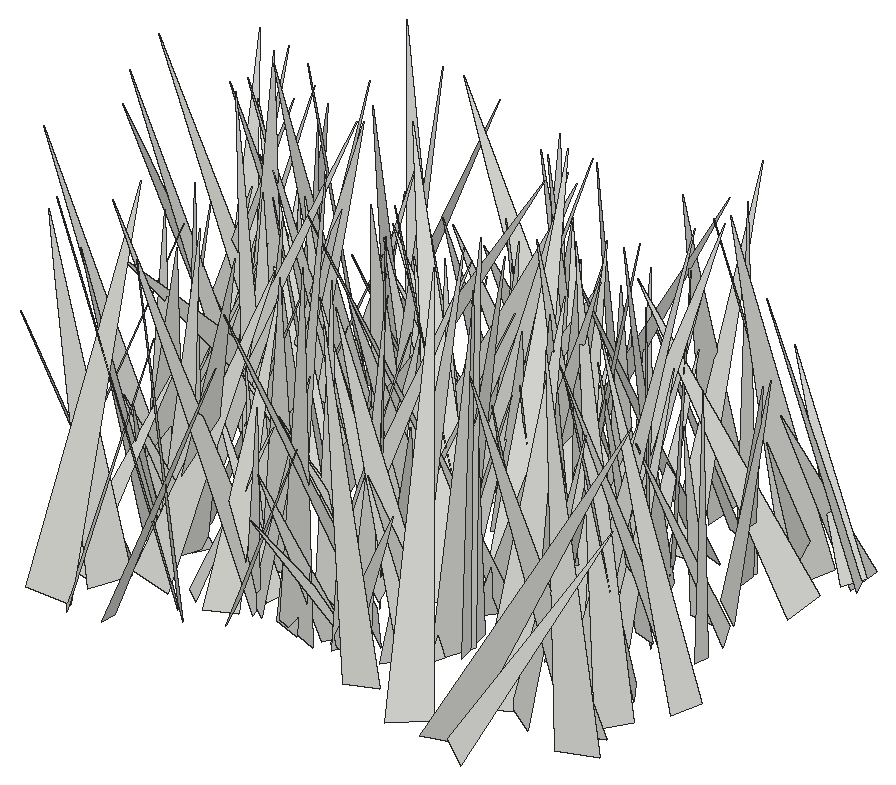
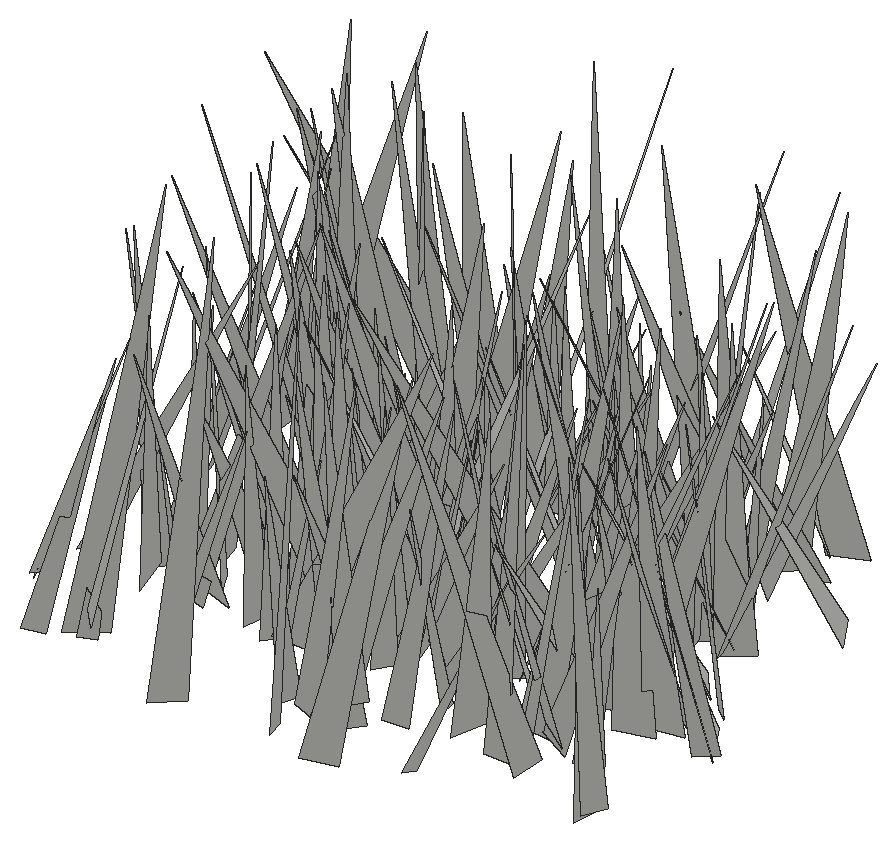
# SketchUp Ruby script. Lengths in inches.
U = 1.inch
M = Sketchup.active_model
def pt(a) = Geom::Point3d.new(a.map { |v| v * U })
def face(e, loops, mat)
  f = e.add_face(loops[0].map { |a| pt(a) })
  loops[1..].each { |l| e.add_face(l.map { |a| pt(a) }).erase! }
  f.material = f.back_material = mat if mat
  f
end
# faces: each face lists its corners as indices into pts; further lists are holes
def faces(e, pts, list, mat = nil) = list.each { |f| face(e, (f[0].is_a?(Array) ? f : [f]).map { |l| l.map { |i| pts[i] } }, mat) }
# xy, xz, yz: faces in a plane at the given z, y or x. An outline is a flat list of corners, or four numbers for a rectangle; further outlines are holes
def ring(l) = l.size == 4 ? [[l[0], l[1]], [l[2], l[1]], [l[2], l[3]], [l[0], l[3]]] : l.each_slice(2).to_a
def flat(e, list, mat, &to3) = list.each { |f| face(e, (f[0].is_a?(Array) ? f : [f]).map { |l| ring(l).map { |u, v| to3.(u, v) } }, mat) }
def xy(e, z, list, mat = nil) = flat(e, list, mat) { |x, y| [x, y, z] }
def xz(e, y, list, mat = nil) = flat(e, list, mat) { |x, z| [x, y, z] }
def yz(e, x, list, mat = nil) = flat(e, list, mat) { |y, z| [x, y, z] }
def lines(e, pts, list) = list.each { |a, b| e.add_line(pt(pts[a]), pt(pts[b])) }
# prism: a flat outline (further loops are holes) pulled along v
def prism(e, loops, v, mat = nil)
  f = face(e, loops, mat); d = Geom::Vector3d.new(v.map { |x| x * U })
  f.pushpull(f.normal.samedirection?(d) ? d.length : -d.length)
end
def box(e, o, s, mat = nil) = prism(e, [[o, [o[0] + s[0], o[1], o[2]], [o[0] + s[0], o[1] + s[1], o[2]], [o[0], o[1] + s[1], o[2]]]], [0, 0, s[2]], mat)
def at(x, y, z, deg = 0) = Geom::Transformation.translation(pt([x, y, z])) * Geom::Transformation.rotation(ORIGIN, Z_AXIS, deg.degrees)
def axes(o, x, y, z) = Geom::Transformation.new([*x, 0, *y, 0, *z, 0, *pt(o).to_a, 1])
def part(name) = M.definitions.add(name)
# library, detail: a bought-in or finely detailed component or shape, given as its bounding box
def library(name, o, s) = part(name).tap { |d| box(d.entities, o, s) }
def detail(e, o, s) = box(e.add_group.entities, o, s)
def put(e, d, t, mat = nil) = e.add_instance(d, t).tap { |i| i.material = mat if mat }
def group(e, t, mat = nil) = e.add_group.tap { |g| g.transformation = t; g.material = mat if mat }.entities
root = M.entities
c1 = part("fur_instance\#9")
p = [[0.8125,0,1.79],[0.67,-0.02,1.48],[0,-0.11,0],[0,0.11,0]]
faces(c1.entities,p,[[0,1,2,3]])
put(root,c1,axes([109.74,45.92,-27.1],[2.70061,4.81345,0.08968],[4.52857,-2.505,-1.92033],[1.63383,-1.01307,5.17446]))
put(root,c1,axes([96.54,47.71,-27.1],[-4.69837,-4.55111,2.1601],[-4.81656,4.92378,-0.10244],[1.47629,1.58022,6.5404]))
put(root,c1,axes([92.45,45.77,-27.1],[-1.03239,7.59334,1.92082],[7.72051,1.31303,-1.04105],[1.31985,-1.74108,7.59215]))
put(root,c1,axes([93.47,47.77,-27.1],[-5.98098,3.27291,2.42019],[3.72115,6.13978,0.89298],[1.64993,-1.98304,6.75918]))
put(root,c1,axes([94.98,45.81,-27.1],[4.77629,1.47467,0.59608],[1.29577,-4.70156,1.24867],[-0.92247,1.03128,4.84029]))
put(root,c1,axes([93.41,45.54,-27.1],[3.76197,3.17485,0.58422],[2.97684,-3.75885,1.25811],[-1.24876,0.60394,4.75913]))
put(root,c1,axes([102.43,50.99,-27.1],[-6.0329,-5.73941,0.68236],[-5.34499,5.91535,2.49841],[2.19943,-1.36753,7.94322]))
put(root,c1,axes([97.98,48.71,-27.1],[5.19096,1.17327,0.15724],[1.14991,-4.82989,-1.92283],[0.28108,-1.90867,4.96239]))
put(root,c1,axes([95.97,48.1875,-27.1],[-5.67662,-5.13617,1.32256],[-5.29359,5.60645,-0.94818],[0.32758,1.59402,7.59639]))
put(root,c1,axes([108.84,46.32,-27.1],[6.56364,-3.25708,1.01889],[-3.38805,-5.95385,2.79299],[0.40967,2.94467,6.77415]))
put(root,c1,axes([100.55,48.92,-27.1],[-1.23371,-7.71978,2.49826],[-7.92295,1.69122,1.31342],[1.75022,2.21429,7.70662]))
put(root,c1,axes([104.48,47.47,-27.1],[-1.23354,6.12021,2.2306],[6.48252,0.93032,1.03231],[-0.63996,-2.37312,6.15735]))
put(root,c1,axes([102.16,49.92,-27.1],[-3.24466,-1.65637,0.06319],[-1.44148,2.88818,1.68993],[0.81834,-1.47993,3.2273]))
put(root,c1,axes([101.77,49.47,-27.1],[1.92833,-3.54748,0.58332],[-3.33012,-2.01195,-1.22706],[-1.35468,-0.10385,3.84674]))
put(root,c1,axes([112.54,49.49,-27.1],[0.14854,-7.36709,1.66817],[-7.40985,-0.46607,-1.39849],[-1.46661,1.60862,7.23466]))
put(root,c1,axes([102.47,48.97,-27.1],[1.15805,-3.96128,0.43832],[-3.70743,-0.90324,1.63219],[1.46246,0.84697,3.79062]))
put(root,c1,axes([113.02,48.37,-27.1],[1.15068,-6.84996,3.27998],[-7.48842,-1.57649,-0.66528],[-1.26644,3.09791,6.914]))
put(root,c1,axes([98.26,49.98,-27.1],[-7.76303,-2.55675,1.09489],[-2.43873,7.81802,0.96517],[1.33728,-0.58482,8.11604]))
put(root,c1,axes([93.29,49.25,-27.1],[-3.10953,-4.00727,0.37973],[-3.98696,3.00024,-0.98706],[-0.55366,0.90108,4.97525]))
put(root,c1,axes([102.33,49.16,-27.1],[3.31226,-1.52366,0.97308],[-1.49474,-3.45052,-0.31491],[-1.01694,0.10903,3.63228]))
put(root,c1,axes([107.26,46.6,-27.1],[5.53383,-2.65462,5.00816],[-4.23304,-6.59023,1.18414],[-3.76962,3.5034,6.0223]))
put(root,c1,axes([92.13,47.67,-27.1],[0.26684,4.21608,0.5662],[4.07293,-0.08948,-1.25314],[1.22767,-0.6195,4.03438]))
put(root,c1,axes([105.17,49.93,-27.1],[4.68158,-4.31782,3.21331],[-4.18207,-5.59908,-1.43065],[-3.3881,0.94493,6.20597]))
put(root,c1,axes([104.95,50.86,-27.1],[4.08531,-1.79648,1.28746],[-1.24322,-4.1049,-1.78292],[-1.82737,-1.22355,4.09124]))
put(root,c1,axes([93.17,50.6,-27.1],[-2.27159,-6.08211,1.19958],[-6.16809,2.34544,0.21162],[0.62109,1.04786,6.48903]))
put(root,c1,axes([110.01,49.09,-27.1],[3.01267,4.99828,1.819],[5.31773,-2.78497,-1.15474],[0.11548,-2.15148,5.72063]))
put(root,c1,axes([94.23,50.82,-27.1],[7.12513,-3.29011,0.44393],[-3.26274,-7.13377,-0.50321],[-0.6135,-0.27186,7.83192]))
put(root,c1,axes([98,49.77,-27.1],[-1.12295,-3.74744,1.45837],[-3.89173,1.39395,0.58526],[1.01223,1.20198,3.86805]))
put(root,c1,axes([94.55,48.62,-27.1],[0.24671,6.36494,1.6516],[6.30189,0.24313,-1.87833],[1.87786,-1.65213,6.08648]))
put(root,c1,axes([96.19,48.82,-27.1],[2.19151,2.85606,0.09461],[2.85445,-2.18225,-0.24214],[0.13471,-0.22234,3.59182]))
put(root,c1,axes([98.43,49.44,-27.1],[2.5994,3.80823,1.24151],[3.99906,-2.55122,-0.54734],[-0.2268,-1.33772,4.57819]))
put(root,c1,axes([91.82,52.03,-27.1],[4.12034,-0.14152,0.59374],[0.17297,-3.61498,-2.06197],[-0.58535,-2.06437,3.57009]))
put(root,c1,axes([94.5625,51.46,-27.1],[1.61464,-3.26071,0.69447],[-2.99454,-1.75765,-1.29032],[-1.46534,-0.00102,3.40211]))
put(root,c1,axes([97.64,48.51,-27.1],[-4.32625,3.6169,1.13686],[3.35652,4.45591,-1.40339],[1.76301,0.39209,5.46158]))
put(root,c1,axes([98.51,50.375,-27.1],[-3.79909,0.62191,0.11225],[0.62576,3.79759,0.13861],[0.08831,-0.15497,3.84716]))
put(root,c1,axes([103.35,48.6875,-27.1],[-6.05732,0.47074,1.68041],[-0.07648,5.99257,-1.95441],[1.74342,1.89841,5.75265]))
put(root,c1,axes([109.24,49.15,-27.1],[-4.71435,5.59524,2.23508],[5.56124,5.13291,-1.11952],[2.31839,-0.93486,7.23039]))
put(root,c1,axes([97.51,51.88,-27.1],[0.93072,-6.54849,1.55591],[-6.7031,-0.75944,0.81335],[0.60996,1.64631,6.5641]))
put(root,c1,axes([100.09,49,-27.1],[3.45024,7.01244,2.07893],[6.95776,-3.8555,1.45774],[-2.25516,-1.1667,7.67811]))
put(root,c1,axes([97.52,50.77,-27.1],[0.08392,3.77547,1.67654],[4.10941,-0.2474,0.35143],[-0.42151,-1.66031,3.76001]))
put(root,c1,axes([105.5625,51.09,-27.1],[7.52534,-2.11015,2.94691],[-2.32099,-8.02168,0.183],[-2.78389,0.98374,7.81345]))
put(root,c1,axes([104.37,49.6,-27.1],[-6.74927,1.80081,2.69667],[1.18797,7.16726,-1.81295],[3.01723,1.2063,6.74602]))
put(root,c1,axes([105.72,51.95,-27.1],[-6.42267,-1.42598,3.31634],[-1.29179,7.22813,0.60623],[3.37087,0.05298,6.55107]))
put(root,c1,axes([91.19,53.39,-27.1],[3.73638,-5.69312,0.32255],[-5.69521,-3.70663,0.54933],[0.28337,0.57053,6.78752]))
put(root,c1,axes([101.1,52.9375,-27.1],[-3.84083,-1.16764,0.10273],[-1.10793,3.73134,0.98769],[0.38264,-0.91633,3.89099]))
put(root,c1,axes([104.73,51.92,-27.1],[7.78387,0.2727,2.09642],[0.3333,-8.05673,-0.18953],[-2.08764,-0.26953,7.78634]))
put(root,c1,axes([100.16,51.05,-27.1],[1.00537,5.49165,1.69021],[5.63183,-1.28199,0.81538],[-1.13911,-1.49133,5.52306]))
put(root,c1,axes([101.02,52.79,-27.1],[5.50119,4.10651,2.99111],[4.73487,-5.74232,-0.82461],[-1.84151,-2.49711,6.81516]))
put(root,c1,axes([89.3,49.86,-27.1],[4.7893,3.01055,0.30481],[2.77693,-4.59952,1.79634],[-1.20208,1.36921,5.36414]))
put(root,c1,axes([93.03,51.84,-27.1],[4.88657,-1.90502,2.44295],[-2.30886,-5.28158,0.49977],[-2.06549,1.39696,5.22091]))
put(root,c1,axes([111.91,52.85,-27.1],[-4.7875,-3.33897,1.34753],[-3.4677,4.87923,-0.23006],[0.96934,0.96392,5.83232]))
put(root,c1,axes([91.79,52.52,-27.1],[0.33576,5.45677,2.6197],[6.05197,-0.25349,-0.24764],[0.11336,-2.62894,5.46148]))
put(root,c1,axes([91.74,53.0625,-27.1],[-7.05109,-1.52018,0.70264],[-1.52291,7.08527,0.04653],[0.69669,0.10238,7.21295]))
put(root,c1,axes([99.61,54.22,-27.1],[-4.59032,-0.23962,0.17171],[-0.16134,4.28449,1.66587],[0.24672,-1.65642,4.28408]))
put(root,c1,axes([113.07,54.03,-27.1],[-6.09562,-2.74651,0.83103],[-2.67616,6.14538,0.68045],[1.03541,-0.28555,6.65108]))
put(root,c1,axes([112.82,50.63,-27.1],[-8.1921,1.36867,0.61461],[1.20152,8.02801,-1.8625],[0.89853,1.74336,8.09413]))
put(root,c1,axes([105.68,54.11,-27.1],[-0.21744,-4.53269,0.61909],[-4.46943,0.07824,-0.99696],[-0.9761,0.65149,4.42703]))
put(root,c1,axes([92.64,53.23,-27.1],[0.05129,-4.93553,2.34933],[-4.99892,0.90807,2.01684],[2.21125,2.16734,4.50493]))
put(root,c1,axes([99.3125,52.04,-27.1],[3.76049,3.04894,0.61025],[2.98388,-3.80785,0.6375],[-0.87456,0.11813,4.79905]))
put(root,c1,axes([99.18,52.47,-27.1],[3.55811,5.92159,0.8478],[5.93377,-3.36884,-1.37307],[0.75783,-1.4247,6.77052]))
put(root,c1,axes([105.36,56.64,-27.1],[1.43301,-8.2393,0.15598],[-8.02359,-1.35888,1.93375],[1.87948,0.48092,8.13635]))
put(root,c1,axes([113.97,53.04,-27.1],[-6.67851,0.63047,0.27765],[0.60623,6.66388,-0.54986],[0.32721,0.52189,6.68563]))
put(root,c1,axes([92.96,52.9,-27.1],[-5.66532,-0.50223,1.85308],[-0.88322,5.80808,-1.12609],[1.70472,1.34012,5.57494]))
put(root,c1,axes([93.61,52.71,-27.1],[4.63443,1.21877,0.59299],[1.09033,-4.6073,0.94811],[-0.80513,0.77609,4.69728]))
put(root,c1,axes([104.89,54.18,-27.1],[7.07738,-3.29601,0.99897],[-3.4049,-7.03943,0.89669],[-0.51794,1.23844,7.75557]))
put(root,c1,axes([100.48,53.51,-27.1],[5.45999,3.37552,0.2587],[3.37248,-5.38033,-0.97518],[0.29572,-0.96459,6.34466]))
put(root,c1,axes([106.65,55.9375,-27.1],[1.50872,-5.62418,0.24688],[-5.60162,-1.47433,0.64555],[0.56049,0.40439,5.78713]))
put(root,c1,axes([99.46,56.03,-27.1],[-0.15941,-4.26775,0.08772],[-3.87813,0.18147,1.78158],[1.78369,0.01316,3.88138]))
put(root,c1,axes([100.71,56.18,-27.1],[1.73584,-5.70606,0.92261],[-5.63591,-1.88469,-1.0526],[-1.28332,0.55882,5.87063]))
put(root,c1,axes([110.05,52.2,-27.1],[3.85814,7.37241,1.12129],[7.37277,-3.96052,0.67189],[-1.11889,-0.67587,8.29374]))
put(root,c1,axes([101.55,57.42,-27.1],[-5.30348,-5.59312,0.1785],[-5.55783,5.29332,0.73008],[0.65218,-0.37354,7.67313]))
put(root,c1,axes([95.92,52.8125,-27.1],[-7.72963,0.57294,0.92033],[0.30078,7.49944,-2.14251],[1.04153,2.08628,7.44883]))
put(root,c1,axes([99.85,54.49,-27.1],[-4.67921,0.76999,0.1435],[0.76372,4.67821,-0.1991],[0.17382,0.17327,4.73796]))
put(root,c1,axes([108.08,53.14,-27.1],[6.4621,3.38539,1.99868],[3.00841,-6.73382,1.67909],[-2.53082,0.63956,7.09931]))
put(root,c1,axes([91.97,52.79,-27.1],[4.66085,6.54813,0.11631],[6.5407,-4.64683,-0.4912],[0.3329,-0.37945,8.02249]))
put(root,c1,axes([93.57,60.04,-27.1],[5.32765,-5.22538,0.29084],[-4.03169,-4.36253,-4.52625],[-3.33686,-3.07194,5.93309]))
put(root,c1,axes([103.35,54.04,-27.1],[-5.00695,6.61488,0.9269],[6.67749,4.92855,0.89773],[-0.16413,-1.27989,8.24744]))
put(root,c1,axes([94.04,57.1,-27.1],[1.95757,-4.55386,0.31612],[-4.56359,-1.94437,0.25034],[0.10577,0.38911,4.95045]))
put(root,c1,axes([102.51,55.01,-27.1],[-0.54447,5.56352,1.73211],[5.79599,0.33809,0.73596],[-0.59958,-1.78391,5.54144]))
put(root,c1,axes([109.8125,55.99,-27.1],[-2.15143,-4.58063,1.63472],[-4.86135,2.07952,-0.57094],[0.14745,1.72526,5.02841]))
put(root,c1,axes([104.61,56.24,-27.1],[-1.9321,-3.03286,0.9193],[-3.13143,1.99261,-0.00754],[0.48737,0.77951,3.596]))
put(root,c1,axes([101.43,56.67,-27.1],[3.99613,2.0991,0.80323],[2.24013,-3.58697,-1.77087],[0.18236,-1.93595,4.15203]))
put(root,c1,axes([109.92,56.12,-27.1],[4.37424,4.04681,2.79179],[4.54542,-4.75288,-0.23239],[-1.87347,-2.08284,5.95454]))
put(root,c1,axes([92.67,57.08,-27.1],[-7.47727,-2.4998,1.10622],[-2.44373,7.5564,0.55783],[1.22512,-0.18436,7.86431]))
put(root,c1,axes([103.01,54.375,-27.1],[-1.19348,5.65379,0.3473],[5.3271,0.99964,2.033],[-1.92561,-0.73875,5.40894]))
put(root,c1,axes([111.91,57.76,-27.1],[-4.09527,-2.1175,0.66115],[-1.87882,4.04889,1.32991],[1.17939,-0.90267,4.41434]))
put(root,c1,axes([93.14,56.36,-27.1],[5.23095,-0.44242,1.6949],[-0.413,-5.49862,-0.16069],[-1.70231,-0.02548,5.24716]))
put(root,c1,axes([90.93,59.19,-27.1],[-1.44964,-7.72306,0.36058],[-7.72764,1.4358,-0.315],[-0.24346,0.41228,7.85162]))
put(root,c1,axes([89.07,56.77,-27.1],[3.62429,3.41254,1.71474],[3.78655,-3.51895,-1.00013],[-0.49783,-1.92166,4.87654]))
put(root,c1,axes([105.39,58.6,-27.1],[5.27759,-3.33069,0.22963],[-3.2336,-5.20637,-1.19863],[-0.83073,-0.89406,6.12452]))
put(root,c1,axes([96.05,56.4,-27.1],[-3.65286,-4.07637,1.60167],[-4.37583,3.48496,-1.11027],[0.18514,1.94004,5.3598]))
put(root,c1,axes([107.84,54.34,-27.1],[0.68594,6.83231,0.78357],[6.74689,-0.82108,1.2531],[-1.33188,-0.64057,6.75135]))
put(root,c1,axes([109.4,55.15,-27.1],[1.25627,4.75609,0.70963],[4.78282,-1.31187,0.32531],[-0.49861,-0.60066,4.90844]))
put(root,c1,axes([104.28,57.26,-27.1],[-2.25784,-3.06403,1.232],[-3.11024,2.47464,0.4545],[1.1102,0.70132,3.77883]))
put(root,c1,axes([100.89,57.57,-27.1],[3.77255,3.78798,3.73229],[4.48771,-4.72284,0.25719],[-2.85294,-2.4201,5.33992]))
put(root,c1,axes([105.02,54.63,-27.1],[-3.53884,7.24303,1.02774],[7.25201,3.62348,-0.56563],[0.96238,-0.67082,8.04145]))
put(root,c1,axes([97.62,57.19,-27.1],[2.40925,-3.29701,1.00546],[-3.44676,-2.29271,0.74099],[0.03277,1.24857,4.01568]))
put(root,c1,axes([112.3,55.95,-27.1],[-4.48133,-0.60292,1.35721],[-0.97091,4.45413,-1.22715],[1.12377,1.44397,4.35201]))
put(root,c1,axes([104.21,58.71,-27.1],[6.83248,-2.68093,1.04491],[-2.55055,-6.88917,-0.99801],[-1.33189,-0.56029,7.27146]))
put(root,c1,axes([100.55,57.34,-27.1],[-3.18222,-1.83698,0.96818],[-1.93012,3.2701,-0.13938],[0.76583,0.60852,3.67173]))
put(root,c1,axes([94.68,54.68,-27.1],[4.61652,6.22378,1.13894],[6.03614,-4.75491,1.51682],[-1.89675,0.0163,7.59914]))
put(root,c1,axes([108.72,58.57,-27.1],[-6.30807,-3.21691,2.7037],[-2.95993,6.86307,1.25992],[2.98285,0.00727,6.96799]))
put(root,c1,axes([101.82,58.65,-27.1],[2.32363,-4.81619,0.47979],[-4.81966,-2.25368,0.71896],[0.44354,0.74187,5.29887]))
put(root,c1,axes([90.77,55.36,-27.1],[3.00596,2.69315,0.13963],[2.45938,-2.82346,1.51258],[-1.10635,1.04086,3.74179]))
put(root,c1,axes([110.53,58.14,-27.1],[0.0054,-4.02258,1.09842],[-4.16704,0.03516,0.14925],[0.15324,1.09787,4.01982]))
put(root,c1,axes([103.375,57.16,-27.1],[3.80415,1.70942,1.42934],[1.7089,-4.05302,0.29902],[-1.42996,-0.29602,4.15984]))
put(root,c1,axes([106.6,56.15,-27.1],[-4.20959,5.12778,0.85898],[5.1677,4.24809,-0.03415],[0.57165,-0.64206,6.63427]))
put(root,c1,axes([105.72,58.4,-27.1],[0.0044,-6.27087,2.13822],[-6.5778,-0.25997,-0.7489],[-0.79272,2.12236,6.226]))
put(root,c1,axes([99.6875,58.52,-27.1],[2.95462,-6.48005,1.02046],[-5.97059,-2.19282,3.36242],[2.71745,2.2277,6.27814]))
put(root,c1,axes([101.51,56.72,-27.1],[2.79902,6.82497,1.56007],[7.00009,-2.70115,-0.74237],[0.11309,-1.72399,7.33919]))
put(root,c1,axes([106.88,56.27,-27.1],[1.72672,7.47142,1.23195],[7.48463,-1.49226,-1.44043],[1.14896,-1.50745,7.53186]))
put(root,c1,axes([96.29,59.34,-27.1],[4.8862,-3.80667,1.31151],[-3.74132,-5.05482,-0.73291],[-1.48774,0.20937,6.1505]))
put(root,c1,axes([105.53,56.51,-27.1],[-3.3116,2.69695,0.72945],[2.42136,3.33487,-1.33716],[1.39378,0.61437,4.05614]))
put(root,c1,axes([91.51,58.28,-27.1],[2.46407,-3.91283,1.91735],[-4.25122,-2.64198,0.07181],[-0.95581,1.66367,4.6235]))
put(root,c1,axes([93.38,58.47,-27.1],[-7.85705,-0.88135,0.16267],[-0.88597,7.85465,-0.23661],[0.1352,0.25331,7.90278]))
put(root,c1,axes([88.35,57.86,-27.1],[3.49532,2.40186,0.16337],[2.40303,-3.46356,-0.49202],[0.14512,-0.49771,4.21237]))
put(root,c1,axes([92.17,58.84,-27.1],[1.0853,-7.02468,2.48253],[-7.23303,-0.3918,2.05344],[1.78669,2.68091,6.80495]))
put(root,c1,axes([110.92,59.05,-27.1],[-1.89095,-4.65132,2.366],[-4.60338,2.67208,1.57395],[2.45798,1.42605,4.76793]))
put(root,c1,axes([96.24,58.22,-27.1],[-6.99068,-2.50094,0.47101],[-2.54423,6.83653,-1.46112],[-0.05835,1.53405,7.27938]))
put(root,c1,axes([87.7,59.31,-27.1],[1.22983,-5.08709,1.30795],[-5.046,-0.77126,1.74491],[1.45845,1.62123,4.93419]))
put(root,c1,axes([95.33,57.26,-27.1],[7.21653,-2.33327,0.39687],[-2.31249,-6.67999,2.77668],[0.50399,2.75925,7.05779]))
put(root,c1,axes([90.52,59.66,-27.1],[1.05516,-7.50337,2.43147],[-7.87164,-0.84629,0.8044],[0.49989,2.51181,7.53438]))
put(root,c1,axes([90.88,55.38,-27.1],[4.07419,5.57288,0.07978],[5.18286,-3.82462,2.48447],[-2.04971,1.40628,6.44076]))
put(root,c1,axes([94.53,57.51,-27.1],[-3.04335,5.85133,0.32291],[5.70958,2.87864,1.64877],[-1.32023,-1.03909,6.38604]))
put(root,c1,axes([110.125,60.67,-27.1],[5.73315,-1.08828,0.33068],[-0.98004,-5.58896,-1.40205],[-0.57725,-1.3198,5.66459]))
put(root,c1,axes([107.92,61.7,-27.1],[-1.99035,-6.59495,0.1128],[-6.59501,1.99173,0.07994],[0.10913,0.08488,6.88828]))
put(root,c1,axes([97.71,59.35,-27.1],[4.40599,-6.63506,1.39046],[-6.52465,-3.70025,3.01783],[1.84021,2.76664,7.37085]))
put(root,c1,axes([92.23,57.55,-27.1],[-0.89857,4.82904,0.37817],[4.8418,0.88433,0.21213],[-0.14006,-0.41036,4.90735]))
put(root,c1,axes([93.55,59.71,-27.1],[3.00214,-3.52749,1.91618],[-3.65397,-3.39209,-0.51969],[-1.66236,1.08552,4.60282]))
put(root,c1,axes([106.88,58.1,-27.1],[2.68485,5.08236,0.90598],[5.15716,-2.6868,-0.21076],[-0.23424,-0.9002,5.74408]))
put(root,c1,axes([87.57,59.23,-27.1],[5.01329,4.55618,1.17415],[4.70331,-4.80639,-1.43108],[0.12753,-1.84671,6.62147]))
put(root,c1,axes([100.75,56.87,-27.1],[4.99959,5.18328,0.38062],[5.01525,-4.9501,1.53324],[-1.36326,0.79826,7.03643]))
put(root,c1,axes([108.39,57.52,-27.1],[-3.90191,2.21296,0.38649],[1.88444,3.64598,-1.85127],[1.22289,1.44261,4.08594]))
put(root,c1,axes([100.03,60.19,-27.1],[-1.04898,-5.12431,2.12616],[-5.35306,1.50327,0.98203],[1.45734,1.83333,5.13756]))
put(root,c1,axes([112.7,60.9375,-27.1],[-6.59727,0.97904,0.29915],[1.02311,6.37288,1.70633],[0.03533,-1.73199,6.44755]))
put(root,c1,axes([103.26,60.07,-27.1],[2.23095,-4.80055,1.901],[-5.14348,-2.24733,0.36107],[-0.45138,1.8816,5.28129]))
put(root,c1,axes([93.06,61.68,-27.1],[-0.40917,-7.70862,1.45343],[-7.84037,0.35495,-0.32469],[-0.25296,1.46762,7.71264]))
put(root,c1,axes([107.66,60.2,-27.1],[5.0794,2.90769,2.21904],[3.29641,-5.28463,-0.62087],[-1.58507,-1.67247,5.81975]))
put(root,c1,axes([103.52,58.44,-27.1],[-5.59441,-0.96055,0.72122],[-1.15543,5.24244,-1.98041],[0.32833,2.08191,5.31959]))
put(root,c1,axes([100.04,59.89,-27.1],[-3.98181,3.20015,0.16473],[3.12043,3.81261,1.36007],[-0.7287,-1.16015,4.92402]))
put(root,c1,axes([99.5625,59.53,-27.1],[-5.02924,-0.94611,0.83871],[-1.10156,4.96734,-1.00192],[0.62059,1.14984,5.01842]))
put(root,c1,axes([89.83,58.93,-27.1],[-1.61925,6.67608,1.38838],[6.8184,1.60284,0.24489],[0.08425,-1.4073,6.86528]))
put(root,c1,axes([89.64,58.07,-27.1],[2.76869,6.15296,0.77217],[6.00563,-2.8712,1.34513],[-1.54517,-0.13446,6.61174]))
put(root,c1,axes([104.3,60.04,-27.1],[1.80379,6.11401,2.80003],[6.29213,-2.55743,1.53087],[-2.37284,-2.13386,6.18799]))
put(root,c1,axes([97.13,57.9,-27.1],[3.53249,6.50702,1.2231],[6.07163,-3.73652,2.34297],[-2.64057,0.11331,7.02355]))
put(root,c1,axes([90.39,62.45,-27.1],[-0.97227,-5.54065,0.71566],[-5.53732,1.05209,0.62249],[0.741,0.5921,5.59077]))
put(root,c1,axes([99.91,61.3,-27.1],[4.11916,-1.93041,1.42636],[-1.9279,-4.34864,-0.31782],[-1.42975,0.30221,4.53795]))
put(root,c1,axes([96.21,61.31,-27.1],[1.60844,-3.68609,1.55705],[-3.78668,-1.94455,-0.69177],[-1.29334,1.10916,3.96179]))
put(root,c1,axes([97.53,61.1875,-27.1],[-2.45268,-3.25533,0.28731],[-3.08329,2.18606,-1.55237],[-1.08306,1.14864,3.76868]))
put(root,c1,axes([103.95,62.06,-27.1],[4.8037,-2.51399,0.9877],[-2.43404,-4.90267,-0.64073],[-1.17095,-0.12226,5.38379]))
put(root,c1,axes([92.3125,59.12,-27.1],[3.84867,2.11329,0.22175],[1.92609,-3.66331,1.48248],[-0.8974,1.20066,4.13285]))
put(root,c1,axes([92.2,61.86,-27.1],[-2.37076,-5.83706,1.32394],[-5.9146,2.06646,-1.48049],[-0.91737,1.76156,6.12372]))
put(root,c1,axes([101.71,60.51,-27.1],[7.5928,-1.32868,0.07278],[-1.31152,-7.40102,1.71058],[0.22497,1.69728,7.51598]))
put(root,c1,axes([93.06,62.25,-27.1],[-4.49464,-4.79472,1.8462],[-5.03521,4.59856,-0.3156],[1.02201,1.56958,6.56442]))
put(root,c1,axes([105.22,61.49,-27.1],[4.42317,-1.03576,2.17466],[-1.28949,-4.85884,0.30856],[-2.03449,0.82776,4.53233]))
put(root,c1,axes([100.25,63.79,-28.22],[2.87814,-5.28951,1.31735],[-4.95416,-3.15966,-1.86304],[-2.27391,0.18887,5.72641]))
put(root,c1,axes([93.09,63.81,-27.1],[-1.97553,-6.78705,1.45707],[-6.65434,2.28292,1.61176],[1.97656,0.90224,6.88251]))
put(root,c1,axes([101.17,61.77,-27.1],[-5.47966,3.19166,2.7493],[3.39794,6.01513,-0.2105],[2.48986,-1.18473,6.33791]))
put(root,c1,axes([94.47,59.96,-27.1],[2.91558,3.30379,0.88214],[2.68077,-2.92801,2.10571],[-2.12289,0.83996,3.8706]))
put(root,c1,axes([97.2,64.09,-27.1],[-0.08674,-5.50292,0.32115],[-5.49794,0.10952,0.39174],[0.3974,0.31411,5.48965]))
put(root,c1,axes([102.82,63.24,-27.1],[-1.51621,-3.26203,0.55212],[-3.23761,1.58793,0.49084],[0.68086,0.28668,3.56354]))
put(root,c1,axes([96.5,62.2,-27.1],[3.55375,0.65284,0.74182],[0.70307,-3.6162,-0.18565],[-0.69441,-0.32026,3.60844]))
put(root,c1,axes([110.43,64.12,-28.22],[6.46231,-4.31648,2.52967],[-3.92803,-6.93665,-1.8017],[-3.09867,-0.20881,7.55958]))
put(root,c1,axes([99.51,63.75,-28.22],[2.89446,-5.47209,0.08006],[-5.31049,-2.7865,1.53693],[1.32243,0.78724,5.99662]))
put(root,c1,axes([92.18,61.76,-27.1],[2.56604,4.25646,1.10853],[4.39439,-2.42581,-0.85772],[0.18887,-1.38883,4.89555]))
put(root,c1,axes([110.15,64.42,-28.22],[4.1039,-1.37964,0.4984],[-1.03776,-3.77714,-1.91052],[-1.03675,-1.68037,3.88527]))
put(root,c1,axes([103.17,61.96,-27.1],[-4.31341,6.46311,1.11663],[6.32564,3.74609,2.75266],[-1.73345,-2.41229,7.26637]))
put(root,c1,axes([89.99,62.39,-27.1],[-3.27969,0.65416,1.38528],[0.68941,3.5533,-0.04576],[1.36808,-0.22237,3.34398]))
put(root,c1,axes([101.04,61.07,-27.1],[4.03542,0.28371,1.50858],[-0.2798,-4.0361,1.5075],[-1.50932,1.50677,3.754]))
put(root,c1,axes([89.51,63.55,-28.22],[5.74214,0.07937,1.80023],[0.34922,-5.94743,-0.85168],[-1.76782,-0.91707,5.67918]))
put(root,c1,axes([98.8125,66.18,-28.22],[5.11337,-4.37567,0.02712],[-4.08728,-4.79107,-2.37351],[-1.56248,-1.78687,6.29758]))
put(root,c1,axes([111.89,65.14,-28.22],[4.14247,-2.36814,0.94959],[-1.79033,-3.98803,-2.13546],[-1.81783,-1.46881,4.26707]))
put(root,c1,axes([109.89,61.37,-27.1],[-6.28866,-0.36775,1.68536],[-0.82762,6.23312,-1.72806],[1.51351,1.8804,6.05775]))
put(root,c1,axes([113.26,63.24,-27.1],[-4.74174,-2.50609,0.51828],[-2.55748,4.67952,-0.77105],[0.09149,0.92453,5.30754]))
put(root,c1,axes([99.17,63.96,-27.1],[4.9839,-2.53795,0.76874],[-2.53211,-5.04073,-0.2255],[-0.78777,0.14572,5.58834]))
put(root,c1,axes([102.23,63.48,-28.22],[3.76138,-1.24538,0.93866],[-1.27843,-3.86595,-0.00634],[-0.89313,0.28885,3.96218]))
put(root,c1,axes([88.23,64.63,-27.1],[6.05752,-0.57817,0.88939],[-0.39,-6.0087,-1.2499],[-0.9865,-1.17476,5.9553]))
put(root,c1,axes([109.7,64.86,-27.1],[-4.76298,-4.61729,1.21885],[-4.61962,4.89113,0.47635],[1.20999,0.49843,6.61653]))
put(root,c1,axes([112.93,63.32,-27.1],[-3.82314,1.91513,0.41484],[1.95484,3.79049,0.51675],[0.13566,-0.64863,4.24466]))
put(root,c1,axes([96.03,64.8,-28.22],[-3.93279,-0.23592,0.50656],[-0.05149,3.7386,1.34138],[0.55643,-1.32147,3.70448]))
put(root,c1,axes([101.16,63.86,-28.22],[1.25077,5.74635,3.18749],[6.40163,-1.79789,0.7292],[-1.48314,-2.91412,5.83551]))
put(root,c1,axes([101.38,65.34,-28.22],[6.5233,2.37968,3.04495],[3.30026,-6.53866,-1.96019],[-2.01069,-3.01183,6.66138]))
put(root,c1,axes([105.36,66.09,-28.22],[7.48346,-2.4752,1.75576],[-1.96533,-7.51292,-2.21472],[-2.31232,-1.62508,7.56464]))
put(root,c1,axes([106.58,65,-28.22],[-1.89303,-4.40404,0.51291],[-4.43222,1.86471,-0.34716],[-0.11875,0.60786,4.78107]))
put(root,c1,axes([91.85,63.7,-27.1],[7.09843,0.26187,0.16049],[0.26265,-7.10014,-0.03187],[-0.15921,-0.03777,7.10319]))
put(root,c1,axes([94.99,62.81,-27.1],[-6.58758,2.43197,1.48528],[2.355,6.75255,-0.6115],[1.60454,0.07391,6.99549]))
put(root,c1,axes([107.4,61.07,-27.1],[1.20703,6.81999,0.05967],[6.70849,-1.19813,1.23829],[-1.22962,0.158,6.81439]))
